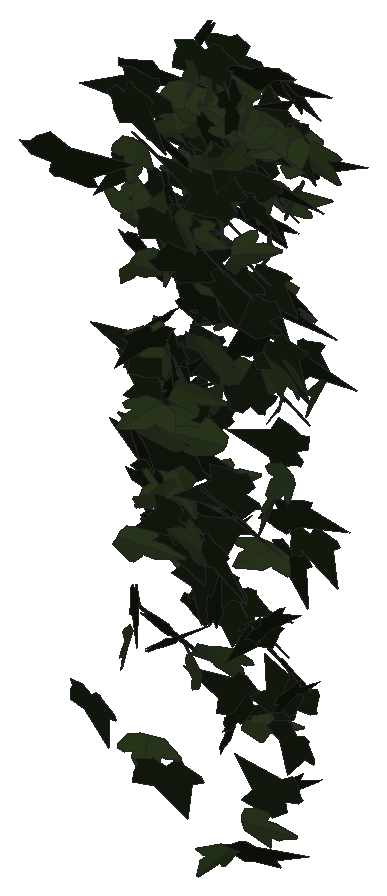
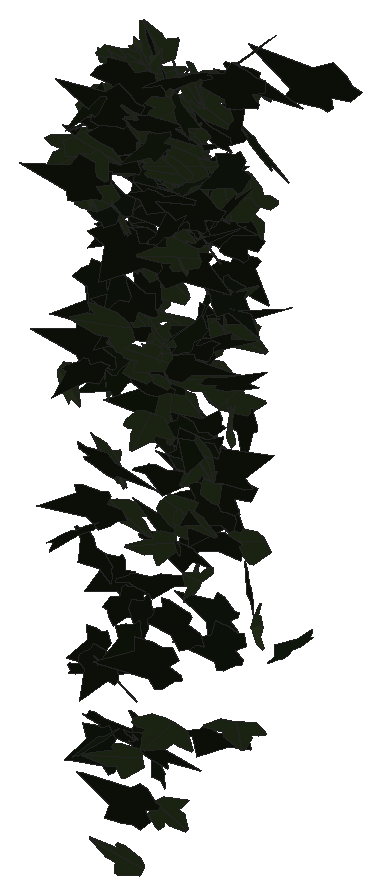
# SketchUp Ruby script. Lengths in millimetres.
U = 1.mm
M = Sketchup.active_model
def pt(a) = Geom::Point3d.new(a.map { |v| v * U })
def face(e, loops, mat)
  f = e.add_face(loops[0].map { |a| pt(a) })
  loops[1..].each { |l| e.add_face(l.map { |a| pt(a) }).erase! }
  f.material = f.back_material = mat if mat
  f
end
# faces: each face lists its corners as indices into pts; further lists are holes
def faces(e, pts, list, mat = nil) = list.each { |f| face(e, (f[0].is_a?(Array) ? f : [f]).map { |l| l.map { |i| pts[i] } }, mat) }
# xy, xz, yz: faces in a plane at the given z, y or x. An outline is a flat list of corners, or four numbers for a rectangle; further outlines are holes
def ring(l) = l.size == 4 ? [[l[0], l[1]], [l[2], l[1]], [l[2], l[3]], [l[0], l[3]]] : l.each_slice(2).to_a
def flat(e, list, mat, &to3) = list.each { |f| face(e, (f[0].is_a?(Array) ? f : [f]).map { |l| ring(l).map { |u, v| to3.(u, v) } }, mat) }
def xy(e, z, list, mat = nil) = flat(e, list, mat) { |x, y| [x, y, z] }
def xz(e, y, list, mat = nil) = flat(e, list, mat) { |x, z| [x, y, z] }
def yz(e, x, list, mat = nil) = flat(e, list, mat) { |y, z| [x, y, z] }
def lines(e, pts, list) = list.each { |a, b| e.add_line(pt(pts[a]), pt(pts[b])) }
# prism: a flat outline (further loops are holes) pulled along v
def prism(e, loops, v, mat = nil)
  f = face(e, loops, mat); d = Geom::Vector3d.new(v.map { |x| x * U })
  f.pushpull(f.normal.samedirection?(d) ? d.length : -d.length)
end
def box(e, o, s, mat = nil) = prism(e, [[o, [o[0] + s[0], o[1], o[2]], [o[0] + s[0], o[1] + s[1], o[2]], [o[0], o[1] + s[1], o[2]]]], [0, 0, s[2]], mat)
def at(x, y, z, deg = 0) = Geom::Transformation.translation(pt([x, y, z])) * Geom::Transformation.rotation(ORIGIN, Z_AXIS, deg.degrees)
def axes(o, x, y, z) = Geom::Transformation.new([*x, 0, *y, 0, *z, 0, *pt(o).to_a, 1])
def part(name) = M.definitions.add(name)
# library, detail: a bought-in or finely detailed component or shape, given as its bounding box
def library(name, o, s) = part(name).tap { |d| box(d.entities, o, s) }
def detail(e, o, s) = box(e.add_group.entities, o, s)
def put(e, d, t, mat = nil) = e.add_instance(d, t).tap { |i| i.material = mat if mat }
def group(e, t, mat = nil) = e.add_group.tap { |g| g.transformation = t; g.material = mat if mat }.entities
root = M.entities
M.materials.add("efeu1").color = [18, 25, 13]
M.materials.add("efeu2").color = [43, 57, 29]
c1 = part("ivyleaf_9")
p = [[39.1,54.8,31.7],[34.5,51.8,30.2],[-5.3,25.2,17.3],[-17.9,28.3,20.9],[-21.6,21.7,17],[-20.2,4.3,5.3],
  [-22.9,-0.3,2.5],[-17.1,-4,-0.6],[-2,-2.1,-1.2],[-0.7,-15.4,-10.1],[16.6,-22.3,-16.7],[21.1,-15.1,-12.5],
  [32.7,-10.7,-11],[46.1,-1.8,-6.6],[30.8,11.2,3.8]]
faces(c1.entities,p,[[0,1,2,3,4,5,6,7,8,9,10,11,12,13,14]],"efeu1")
c2 = part("ivyleaf_10")
p = [[0,12.8,-0.8],[-1.5,51.3,-10.9],[-4.9,51,-11.6],[-13.6,26.5,-7.3],[-13.2,15.9,-4.6],[-21.1,19.3,-7.2],
  [-29.5,16.3,-8.3],[-29.2,8.3,-6.2],[-19.7,-9.8,0.5],[-7.6,-13,4],[1,-12.2,5.8],[-0.4,51.1,-11.1],
  [-1.5,51.1,-10.9],[1,-12.4,5.9],[16.9,-12.4,3.5],[35.1,9.1,-5.1],[35,12.9,-6.1],[20.5,16.4,-4.9],
  [15.8,15,-3.8],[15.3,27.6,-7.1],[12.8,31.3,-7.8]]
faces(c2.entities,p,[[0,1,2,3,4,5,6,7,8,9,10],[11,12,0,13,14,15,16,17,18,19,20]],"efeu2")
put(root,c1,axes([3472.1,793,1622],[-0.35225,-0.18046,-0.9132],[-1.40311,-0.54002,0.25614],[-1.0816,0.75932,-0.03487]))
put(root,c1,axes([3451.8,772.5,1506.4],[-1.43595,0.46546,-0.42029],[0.62665,-0.2656,-0.88522],[-1.01583,-0.8218,0.04804]))
put(root,c2,axes([3421.8,859.5,1058.3],[-0.14393,0.1182,1.04111],[1.12553,-0.85686,0.14023],[1.64618,0.59618,-0.00486]))
put(root,c1,axes([3420.9,714,625.1],[0.19793,-0.92787,0.30072],[0.10417,-0.29639,-0.93345],[1.85342,0.11575,0.02035]))
put(root,c1,axes([3419,841,1495.8],[1.48979,-0.40489,-0.12318],[-0.20728,0.05755,-0.88129],[0.77832,0.79032,0.00107]))
put(root,c2,axes([3427.2,791.4,692.5],[0.34181,-0.37409,0.90819],[0.86577,-0.78658,-0.41396],[1.65679,0.48821,0.02895]))
put(root,c1,axes([3446.5,854.7,1412.6],[-0.36434,-0.24057,0.98515],[-0.90275,-0.86488,-0.30337],[1.70589,-0.50907,0.04986]))
put(root,c1,axes([3442.7,959.7,1644.3],[-0.86292,0.18215,-0.71547],[0.99799,-0.5116,-0.46255],[-0.98914,-0.67509,0.15749]))
put(root,c1,axes([3405,648.6,1545.1],[0.13222,-0.03569,1.15238],[2.04046,-0.42261,-0.07772],[0.80705,1.07434,0.00771]))
put(root,c1,axes([3455.6,781.9,1041.6],[0.91727,-0.17025,-0.85565],[-1.54105,0.27662,-0.51113],[0.61813,0.94229,-0.00455]))
put(root,c2,axes([3440.8,786.4,1418.5],[1.79924,0.10195,-0.02577],[0.04852,0.00397,0.95086],[0.19417,-0.94572,0.00121]))
put(root,c2,axes([3459.5,906.5,1051.1],[1.15014,-0.60497,-0.52342],[-0.65175,0.39721,-0.85447],[1.37596,0.69383,0.03278]))
put(root,c1,axes([3450.8,902.9,1064.1],[0.50747,0.81799,0.29214],[0.15403,0.28087,-0.8603],[-1.64591,0.27849,0.00956]))
put(root,c1,axes([3414.8,862.5,690.6],[1.31175,-0.47271,0.40824],[0.64514,-0.22753,-0.83576],[0.99844,0.76808,0.00367]))
put(root,c1,axes([3480.1,836.1,968.6],[0.39127,-0.112,1.07152],[-1.82011,0.48333,0.23401],[-0.94415,-0.97816,-0.00706]))
put(root,c1,axes([3452.8,976.5,1432.7],[-0.56216,-0.50969,0.66162],[0.75309,0.53261,0.58696],[-1.39979,0.49124,0.05008]))
put(root,c1,axes([3425.8,943.7,1249.7],[0.47858,-0.74354,0.48384],[0.268,-0.46307,-0.7848],[1.66692,0.28792,-0.01273]))
put(root,c1,axes([3414.9,825.1,1621.7],[0.88499,-0.05133,0.75556],[1.4328,-0.06475,-0.46773],[0.15619,0.88482,0.0096]))
put(root,c1,axes([3474.7,820.2,1102.8],[-1.25047,-0.63451,-0.00932],[-0.01096,-0.00745,0.9134],[-1.20768,0.65706,0.00135]))
put(root,c2,axes([3421.9,806.3,847.5],[-0.4665,-0.16136,-0.92547],[1.69703,0.26113,-0.28169],[0.56284,-0.92108,0.08227]))
put(root,c1,axes([3437.2,795.7,766.4],[-0.46223,0.12383,-0.9645],[1.62416,-0.44946,-0.27259],[-0.88726,-0.88726,0.00348]))
put(root,c1,axes([3451.5,901.8,1031.2],[-0.84074,-0.25168,0.71456],[1.18175,0.35361,0.50842],[-0.82604,0.76204,0.00008]))
put(root,c1,axes([3420.4,930.4,1453.5],[0.41714,-0.14525,0.87945],[1.61546,-0.24247,-0.25159],[0.5179,0.87332,0.07642]))
put(root,c2,axes([3456.2,884.2,1011.5],[-0.35114,-0.51425,-0.85622],[0.43905,0.82522,-0.54534],[1.84948,-0.29354,-0.0331]))
put(root,c2,axes([3451.9,974.7,595.6],[-1.63447,-0.09893,-0.32733],[0.61837,0.03983,-0.86448],[0.20293,-0.9182,-0.00224]))
put(root,c2,axes([3454.8,801.4,521.4],[1.43667,0.49216,-0.09203],[-0.14734,-0.04977,-0.90114],[-0.94145,0.75883,0.00059]))
put(root,c1,axes([3471.4,884.9,1370],[0.04755,-0.78714,-0.50493],[0.03315,-0.50463,0.78754],[-1.77951,-0.03043,0.00118]))
put(root,c2,axes([3470.4,836,943.6],[-0.47796,-0.40608,0.90458],[-0.16294,-0.92078,-0.43712],[1.88007,-0.18303,0.19208]))
put(root,c1,axes([3456.2,871,1371.3],[-0.58123,0.7564,0.28371],[0.04531,-0.29475,0.81146],[1.53685,0.29476,0.08337]))
put(root,c2,axes([3465.2,809.5,1397.4],[-1.28858,-0.9214,-0.03429],[-0.0056,-0.04039,1.14321],[-1.75482,0.67672,0.02153]))
put(root,c1,axes([3449.3,919.6,1491.4],[0.22992,-0.88095,0.22752],[0.10537,-0.22197,-0.88887],[1.72843,0.13072,0.02392]))
put(root,c2,axes([3442.8,936.6,1382.9],[0.20751,0.1087,0.91296],[1.09784,0.70781,-0.15317],[-1.36257,0.58685,0.01563]))
put(root,c2,axes([3462.6,923.6,1361.1],[1.0144,-0.74913,-0.00724],[0.01572,-0.00301,0.91938],[-1.42572,-0.53304,0.00499]))
put(root,c1,axes([3497.8,780.3,1191],[-0.87149,-0.83133,-0.32685],[-0.31015,-0.28339,0.94908],[-1.67155,0.48601,-0.00569]))
put(root,c2,axes([3466.2,875.3,795.8],[0.3753,0.516,-0.72589],[0.41139,0.69351,0.5517],[1.64432,-0.29128,0.02765]))
put(root,c1,axes([3471.9,853.8,1394.2],[-1.33431,-0.74002,-0.23058],[0.30808,0.16426,-1.01938],[1.44266,-0.71952,0.00443]))
put(root,c1,axes([3461.9,828,907.5],[0.89835,0.56869,0.60064],[0.68281,0.48236,-0.73864],[-1.41844,0.59237,0.02484]))
put(root,c1,axes([3496.5,973.7,1610.7],[-1.50219,-0.25026,0.31227],[-0.57647,-0.07768,-0.82786],[0.49774,-0.84526,-0.01637]))
put(root,c1,axes([3511.1,964,544.1],[-1.08883,-0.13817,-0.71312],[-1.32084,-0.16401,0.58855],[-0.40813,0.89941,-0.00223]))
put(root,c1,axes([3456.4,977.5,1588.7],[1.25013,-0.51269,-0.28318],[-0.27366,0.27133,-0.82475],[1.08059,0.66184,0.11875]))
put(root,c1,axes([3488.3,789.8,1248],[-0.58696,0.77516,-0.55379],[0.3898,-0.51452,-0.83426],[-1.7707,-0.37022,-0.00008]))
put(root,c1,axes([3443.6,797.7,1339],[0.41083,-0.30888,0.92443],[0.93141,-0.78447,-0.37639],[1.60419,0.53457,-0.0182]))
put(root,c1,axes([3491.7,895.4,1339.6],[-0.00193,0.24337,-0.98585],[-0.07847,-0.98505,-0.24313],[-1.931,0.03979,0.01087]))
put(root,c1,axes([3496.1,824.6,1162.6],[-0.80452,-0.31573,0.75062],[-1.05369,-0.50875,-0.52579],[1.1365,-0.69519,0.04388]))
put(root,c1,axes([3486,809.7,1524],[1.089,-0.74475,0.46475],[-0.49561,0.38579,0.93883],[-1.59555,-0.62814,0.02558]))
put(root,c2,axes([3485.6,906.9,1545],[-0.05226,0.65443,0.5911],[-0.0415,-0.59171,0.65409],[1.67784,0.00575,0.03459]))
put(root,c1,axes([3474,828.9,901],[1.3801,0.61982,-0.03086],[-0.04688,-0.01867,-0.95395],[-1.18018,0.72556,0.00181]))
put(root,c2,axes([3463,961,898.1],[0.03235,-0.05018,-0.93059],[1.1374,0.71476,-0.02763],[1.36097,-0.59615,0.04521]))
put(root,c2,axes([3490.2,912.7,1410.8],[1.3228,-0.55146,-0.36174],[-0.46281,0.27423,-0.88527],[1.16676,0.73399,0.05897]))
put(root,c1,axes([3508.2,896,1158.9],[-0.40564,-0.42032,-0.7923],[-0.53349,-0.74235,0.46923],[-1.62144,0.3494,0.04382]))
put(root,c2,axes([3473.9,752.6,1352.7],[-0.56934,-0.50266,-0.84866],[0.82035,0.73105,-0.58494],[1.68849,-0.52467,-0.00197]))
put(root,c2,axes([3504.5,935.2,1220.5],[0.52954,-0.21537,0.86431],[-1.3157,0.5188,0.35182],[-1.06904,-0.74518,-0.00486]))
put(root,c1,axes([3484.1,923.8,1222.8],[-0.42192,-0.61773,0.64797],[-0.42322,-0.60862,-0.6563],[1.65043,-0.31399,-0.00265]))
put(root,c1,axes([3489,803.2,1464.5],[0.72836,-0.26813,-0.83036],[-1.26472,0.49808,-0.4671],[1.07628,0.76674,0.01305]))
put(root,c1,axes([3477.3,858.6,1032.8],[-0.55077,-0.1796,0.92444],[1.42571,0.54216,0.33984],[-1.08613,0.80274,-0.02269]))
put(root,c2,axes([3496.9,781.1,1216.3],[-0.12586,0.54344,0.78565],[-0.26002,-0.78482,0.53136],[1.79941,-0.07539,0.13174]))
put(root,c2,axes([3483,790.9,938.4],[-0.84604,-0.82706,0.12784],[0.11572,0.11246,0.93895],[-1.58854,0.44867,0.00031]))
put(root,c1,axes([3469,739.4,1638.1],[0.74444,-0.94154,-0.38299],[-0.27324,0.35508,-1.01955],[1.91513,0.41665,0.00341]))
put(root,c2,axes([3520.4,871.1,901.2],[-0.70942,-0.02316,0.83819],[-1.55841,-0.18747,-0.36932],[0.34366,-0.89797,0.05549]))
put(root,c1,axes([3444.3,829.3,927],[0.6763,-0.23544,1.06071],[1.59742,-0.6492,-0.42528],[1.31314,0.911,-0.02894]))
put(root,c2,axes([3485.9,783.9,1054.6],[-1.99103,0.01951,0.22966],[0.43523,-0.04542,1.04556],[0.05478,1.0701,0.04019]))
put(root,c2,axes([3459.2,906.7,1519.4],[0.69793,0.14062,0.84622],[1.32736,0.48695,-0.38315],[-0.95055,0.78323,0.08629]))
put(root,c1,axes([3472.7,845,863.6],[-0.90683,-0.33009,-0.79839],[1.22799,0.47036,-0.57954],[1.09342,-0.80201,-0.01129]))
put(root,c1,axes([3473.7,905.6,1402.5],[1.48046,-0.44693,-0.23945],[-0.36978,0.1423,-0.89676],[0.89133,0.80136,0.02569]))
put(root,c1,axes([3481.2,940.5,1472],[-0.86592,-0.61852,-0.52069],[0.60132,0.41394,-0.7678],[1.41639,-0.55387,0.00764]))
put(root,c2,axes([3505,870.1,879.7],[0.05304,-0.00437,-0.91531],[-0.91449,-0.77948,-0.01091],[-1.48271,0.48061,-0.02601]))
put(root,c2,axes([3515.6,824.8,1574.3],[-0.8509,-0.61172,0.73961],[-0.82835,-0.59798,-0.75769],[1.62808,-0.62396,0.00104]))
put(root,c1,axes([3475.5,797.9,692.6],[0.34244,0.8728,-0.18622],[0.03602,0.18619,0.89095],[1.69811,-0.17996,0.01866]))
put(root,c1,axes([3460.1,965.9,693.1],[1.33731,0.06434,0.59038],[1.12238,0.03219,-0.70541],[-0.13321,0.91719,-0.01665]))
put(root,c2,axes([3513.3,861.8,1476.4],[-0.09066,-0.01804,-0.91004],[-1.21842,-0.64713,0.04634],[-1.23143,0.64162,0.02115]))
put(root,c1,axes([3526.9,875.8,1444.9],[-1.23225,0.34529,0.47022],[-0.82631,0.18399,-0.73293],[-0.74159,-0.77876,0.03533]))
put(root,c1,axes([3462.8,930.8,1444.9],[1.40363,-0.49471,0.29596],[0.46353,-0.16819,-0.88805],[0.99443,0.77667,-0.0038]))
put(root,c2,axes([3505.3,844.2,1636.3],[0.60606,-0.72157,-0.55667],[-0.40953,0.51347,-0.78867],[1.68542,0.38423,0.00854]))
put(root,c2,axes([3472.2,885,1445.5],[1.5058,-0.07752,-0.50345],[0.96452,0.02601,0.79243],[-0.09776,-0.93743,0.06362]))
put(root,c1,axes([3487.4,843.5,1536.7],[-1.24516,0.53903,0.58756],[0.82009,-0.40048,0.84721],[1.27686,0.78287,0.02883]))
put(root,c2,axes([3496.6,878.6,1537],[-0.74562,-0.68563,-0.50952],[0.48997,0.43972,-0.78966],[1.55017,-0.46877,0.00451]))
put(root,c1,axes([3494.5,906,1022.5],[-0.62724,0.92555,0.04367],[0.02648,-0.0414,0.98248],[1.76327,0.32987,0.00078]))
put(root,c2,axes([3505.2,892.3,1090.4],[-0.5695,-1.00001,-0.37227],[0.16506,0.36256,-1.04363],[2.02409,-0.31093,-0.01964]))
put(root,c1,axes([3508.6,919.9,490.5],[0.0511,0.27281,0.86951],[0.29972,0.85541,-0.27325],[-1.7083,0.15824,-0.02193]))
put(root,c2,axes([3507.8,840.5,1333.3],[0.12143,-1.03745,0.12459],[0.00582,-0.12463,-1.0394],[1.98865,0.06371,-0.00457]))
put(root,c1,axes([3514.3,738.3,1257.3],[-0.21622,0.57953,-0.79444],[0.35502,-0.7725,-0.5902],[-1.83754,-0.21744,-0.02055]))
put(root,c2,axes([3501.3,955.6,1091.2],[-0.89499,-0.68373,-0.44092],[0.48793,0.35879,-0.82981],[1.46949,-0.53556,0.00699]))
put(root,c2,axes([3510.6,921.9,1208],[-0.05726,-0.04578,0.92637],[-0.06297,-0.92622,-0.04684],[1.7641,-0.03455,0.0284]))
put(root,c2,axes([3493,902.4,1601.4],[-1.50446,0.02593,-0.4214],[0.80106,-0.02151,-0.79089],[-0.06281,-0.89554,0.00679]))
put(root,c1,axes([3493.1,799.5,493],[-0.63446,-0.6476,-0.54356],[0.47618,0.48255,-0.72836],[1.53704,-0.41681,0.00128]))
put(root,c1,axes([3491.6,893,1649.6],[-0.23988,-1.01416,-0.28006],[0.18337,0.26975,-1.02019],[1.99397,-0.14681,0.06013]))
put(root,c1,axes([3514.6,896.5,1417.8],[0.21009,-0.57035,-0.66871],[0.23863,-0.65685,0.58094],[-1.65562,-0.16705,-0.00113]))
put(root,c2,axes([3501.6,716,1570.2],[1.51618,-0.51106,0.18272],[0.29656,-0.09549,-0.94648],[0.98945,0.81174,0.00369]))
put(root,c1,axes([3519,791.2,922.7],[-0.57672,-0.32577,0.79941],[-0.83181,-0.67272,-0.43982],[1.41678,-0.52757,0.06719]))
put(root,c2,axes([3508.3,831.7,1617.6],[1.23757,0.89956,-0.27856],[-0.35084,-0.21038,-1.10968],[-1.75757,0.6754,0.02537]))
put(root,c1,axes([3515.5,849.3,1388.6],[1.27885,0.09743,-0.58653],[-1.11599,-0.03779,-0.67805],[-0.18714,0.89112,0.03537]))
put(root,c2,axes([3525,731.2,1136.9],[1.01914,0.45469,-0.69958],[-1.06461,-0.42114,-0.70188],[-1.17822,0.77383,0.02908]))
put(root,c1,axes([3477.5,896.5,727.8],[0.25697,-0.0047,-0.9318],[1.70179,0.26557,0.12823],[0.49898,-0.90331,0.04255]))
put(root,c2,axes([3484,912.2,1500.6],[1.03521,-0.13561,-0.83686],[1.58512,-0.10017,0.55757],[-0.30127,-0.99306,0.05804]))
put(root,c2,axes([3491.4,947,1196.2],[0.47382,0.06479,-0.89605],[1.60611,0.30203,0.25631],[0.58641,-0.87958,0.022]))
put(root,c2,axes([3516.8,784.4,1370.2],[1.09888,-0.69903,0.28494],[0.34884,-0.21818,-0.90665],[1.39368,0.60578,0.00227]))
put(root,c2,axes([3557.3,868.8,1526.8],[0.5791,0.05979,-0.98206],[-1.86847,0.08596,-0.29895],[0.12298,1.02451,0.08239]))
put(root,c1,axes([3482.6,854.7,998.8],[1.08815,0.01164,-0.82271],[1.49859,0.28289,0.55122],[0.45428,-0.9611,0.15229]))
put(root,c1,axes([3532.6,918.5,535.4],[-0.80314,0.62784,-0.45369],[-0.57397,0.34272,0.75478],[1.35792,0.5162,0.0507]))
put(root,c1,axes([3510.2,776.5,1434.4],[-0.0815,-0.8497,-0.56476],[0.09102,0.56297,-0.85063],[1.93964,-0.06212,0.01619]))
put(root,c1,axes([3545.9,861.2,1408.2],[-1.22915,0.58215,-0.09351],[0.13312,-0.06207,-0.86948],[-1.11423,-0.64961,-0.00072]))
put(root,c1,axes([3518.6,776.5,1151.3],[0.28519,0.25189,1.10714],[1.10666,0.94216,-0.29306],[-1.85609,0.60045,-0.00462]))
put(root,c1,axes([3511,847,1176.8],[-0.07456,-0.50955,-0.87742],[0.21257,0.87058,-0.51056],[1.91935,-0.11621,0.02246]))
put(root,c2,axes([3517.1,854.5,1620],[1.2651,-0.68417,0.48045],[0.63147,-0.34751,-0.9539],[1.46044,0.74292,-0.00374]))
put(root,c2,axes([3496.6,861.9,1553.2],[1.04427,0.18477,0.81134],[1.42252,0.3177,-0.57783],[-0.69604,0.9265,0.03634]))
put(root,c2,axes([3502.1,778.8,1203.1],[-0.14878,0.06743,1.06056],[1.64322,-0.61598,0.1028],[1.1792,0.86688,-0.00945]))
put(root,c2,axes([3526.5,951.7,1596.8],[1.67257,-0.18659,0.06142],[0.11548,-0.00995,-0.89841],[0.35559,0.88091,0.00286]))
put(root,c2,axes([3519,872.9,1603.8],[1.48686,-0.3259,0.37248],[0.68454,-0.10427,-0.84561],[0.64705,0.85919,0.03867]))
put(root,c2,axes([3511.8,807.8,1397.2],[-1.08252,-0.29266,-0.91905],[1.51329,0.46167,-0.6391],[1.03907,-0.97726,-0.02669]))
put(root,c2,axes([3502.7,788.2,1084.9],[-0.56446,-0.13942,-1.02034],[1.89134,0.23974,-0.32162],[0.51406,-1.03517,0.06294]))
put(root,c1,axes([3520.9,791.9,1208.2],[0.54938,-0.38591,-0.95824],[1.36157,-0.64305,0.47449],[-1.41827,-0.76683,0.08434]))
put(root,c1,axes([3528.9,866.4,849],[-0.14633,0.89712,0.18789],[0.00572,-0.1883,0.90031],[1.74442,0.07587,0.01281]))
put(root,c2,axes([3514.4,800.1,986],[1.04204,-0.25034,0.82787],[1.38422,-0.39694,-0.60105],[0.89075,0.90971,-0.03444]))
put(root,c1,axes([3534.4,941.1,1374.9],[1.83949,0.27053,-0.15593],[-0.28598,-0.04166,-1.00367],[-0.52094,0.97813,0.00038]))
put(root,c2,axes([3525.4,890.3,1130.5],[0.33883,-0.28673,-0.85954],[0.91901,-0.71119,0.33726],[-1.45921,-0.51449,0.01282]))
put(root,c1,axes([3531.2,942.2,703.1],[1.45417,-0.44787,-0.24673],[-0.3856,0.14215,-0.88544],[0.89352,0.79023,0.01944]))
put(root,c1,axes([3570.5,786.6,1287.5],[0.37655,-0.16216,0.92337],[-0.8184,0.82289,0.23665],[-1.58549,-0.46327,0.09715]))
put(root,c2,axes([3544.4,838.9,1532.3],[-0.17512,-0.36241,-0.93936],[0.58513,0.88811,-0.37276],[1.8247,-0.31957,0.02938]))
put(root,c1,axes([3545.5,819.3,1593.5],[0.81087,-0.45107,-0.65872],[-0.87628,0.47115,-0.62042],[1.2413,0.62726,-0.00767]))
put(root,c2,axes([3518.7,863.1,1269.3],[0.44042,-0.21025,-0.99383],[1.42272,-0.65492,0.31261],[-1.30906,-0.78252,0.00539]))
put(root,c1,axes([3553.5,841.9,816.8],[-1.61427,-0.26055,-0.44335],[0.80352,0.13541,-0.88729],[0.55877,-0.94744,-0.00489]))
put(root,c1,axes([3584.3,826.4,1464.8],[-1.26834,-0.74334,-0.28833],[-0.37624,-0.21001,0.99832],[-1.47005,0.69509,-0.00673]))
put(root,c2,axes([3516.9,785.4,1145.5],[-0.54297,-0.09337,1.02708],[1.93938,0.13859,0.29565],[-0.30228,1.05692,0.05196]))
put(root,c2,axes([3528.1,962.5,511.8],[-0.07738,-0.07681,-0.92279],[1.47689,0.50114,-0.0759],[0.96155,-0.77591,0.04232]))
put(root,c2,axes([3522.7,968.4,337.9],[0.2469,-0.0419,-0.87246],[1.54196,-0.32381,0.13602],[-0.62116,-0.82046,-0.00913]))
put(root,c1,axes([3536.1,907.8,1257.6],[0.04499,-0.21488,0.90008],[0.33805,-0.88258,-0.21537],[1.72842,0.17821,0.01869]))
put(root,c1,axes([3529.3,926,731.5],[0.5796,-0.14624,-0.91366],[1.56261,-0.40083,0.33783],[-0.81205,-0.8757,-0.00205]))
put(root,c2,axes([3565.7,840.9,359.2],[-0.42544,-0.67295,0.54403],[-0.2041,-0.53601,-0.70709],[1.63423,-0.24213,0.05332]))
put(root,c2,axes([3565.1,835.5,1405.5],[0.14805,-0.18076,-0.96008],[-0.21675,0.95487,-0.18901],[1.84665,0.12657,0.05479]))
put(root,c1,axes([3554.8,880.3,773],[-0.98627,-0.83814,-0.24813],[0.27427,0.20259,-0.98528],[1.64081,-0.53766,0.01554]))
put(root,c1,axes([3544,939.1,1226.2],[-0.0974,-0.60134,-0.66443],[0.3498,0.64432,-0.5973],[1.66928,-0.17011,0.0864]))
put(root,c1,axes([3564.1,910.7,1638.6],[1.05893,0.71118,-0.20448],[-0.24967,-0.15698,-0.90294],[-1.38604,0.57161,0.00643]))
put(root,c1,axes([3544.5,928.7,1253.7],[1.59945,0.36729,0.12652],[-0.23822,-0.02944,0.91687],[0.6999,-0.84936,0.02294]))
put(root,c1,axes([3550.1,912.2,1428.5],[0.93371,-0.7094,-0.43293],[-0.41179,0.37637,-0.86191],[1.52715,0.53522,0.03228]))
put(root,c1,axes([3602.5,958.5,994.3],[-1.07119,0.31778,0.65359],[-1.07659,0.32745,-0.64633],[-0.86837,-0.79796,-0.00494]))
put(root,c2,axes([3589.1,785,1080],[0.27304,0.2623,0.92207],[-0.94673,-0.77663,0.29832],[1.55966,-0.51734,0.01966]))
put(root,c1,axes([3545.2,934,1545.7],[1.53374,0.55117,0.07252],[-0.16469,-0.00178,0.97519],[1.04514,-0.80913,0.04725]))
put(root,c1,axes([3563.1,831.8,928.7],[-1.06235,-0.56935,-0.43165],[0.56127,0.31533,-0.79728],[1.23856,-0.63124,-0.00895]))
put(root,c2,axes([3568.9,842.2,1283.8],[-0.97383,-0.80094,-0.39216],[0.41997,0.32436,-0.95037],[1.64448,-0.55714,0.01047]))
put(root,c1,axes([3567.1,855.8,1535.2],[-0.77059,-0.86177,0.12051],[-0.06161,-0.11791,-0.95193],[1.65494,-0.40566,0.02068]))
put(root,c2,axes([3572.1,938.9,1416.4],[0.95106,-0.75757,0.09475],[0.11311,-0.0743,-0.90749],[1.44862,0.50316,0.00865]))
put(root,c2,axes([3570.3,772,692.5],[-0.79677,0.68437,0.57434],[0.49206,-0.51433,0.80132],[1.62763,0.4905,0.0389]))
put(root,c1,axes([3543.6,873.8,1556.2],[0.02093,-0.07092,-0.97432],[1.2312,0.73065,-0.04588],[1.39316,-0.64465,0.05518]))
put(root,c2,axes([3547.1,971.5,1243.6],[-0.86134,0.17463,-0.92439],[1.63326,-0.34364,-0.48507],[-0.73355,-0.97017,0.00542]))
put(root,c2,axes([3560.8,751.6,1450.3],[-0.19825,0.22538,-1.01255],[0.7487,-0.93304,-0.24815],[-1.82677,-0.40686,0.00818]))
put(root,c1,axes([3610.8,813.9,1636.1],[-0.26707,0.02184,-1.08873],[-1.90547,0.42913,0.13765],[0.81508,1.01038,-0.03493]))
put(root,c2,axes([3595.2,844.1,1596.3],[-1.01927,0.90235,-0.1716],[-0.2355,0.12595,1.04848],[1.73219,0.54809,0.04157]))
put(root,c2,axes([3584.6,857,1292.8],[0.03798,0.20091,-0.85382],[-0.33471,-0.83578,-0.20077],[-1.63547,0.17572,0.02126]))
put(root,c2,axes([3604.3,835.5,1585.7],[0.76625,0.49015,0.7051],[-0.89315,-0.52658,0.63402],[1.36868,-0.61804,0.01899]))
put(root,c1,axes([3561,741.6,1377.3],[-0.1751,-0.05453,1.03704],[1.90886,0.26521,0.10292],[-0.51233,1.00676,0.02905]))
put(root,c1,axes([3590.2,789.9,785.8],[-0.20763,-0.2453,0.88445],[0.65113,0.81562,0.26841],[-1.62095,0.35905,-0.00547]))
put(root,c1,axes([3564.9,947.6,1420.1],[1.3549,-0.36236,-0.50729],[0.8679,-0.22236,0.79879],[-0.80902,-0.84541,0.00734]))
put(root,c1,axes([3553.3,954.7,1595.4],[0.53239,-0.26078,0.81831],[1.49597,-0.26908,-0.35445],[0.65871,0.82187,0.1436]))
put(root,c2,axes([3597.5,902.1,1347.8],[-0.00335,-0.61601,-0.92274],[-0.01581,0.92272,-0.61598],[2.11148,0.00593,-0.00608]))
put(root,c2,axes([3615.1,845,1185],[-1.26371,-0.45428,0.51951],[-0.76258,-0.3332,-0.80348],[1.06937,-0.77444,0.04095]))
put(root,c1,axes([3601.7,890.5,726.1],[-0.16792,0.2841,-0.87622],[0.45006,-0.84375,-0.29738],[-1.69434,-0.25228,0.00785]))
put(root,c1,axes([3604.4,921.1,1540.6],[-1.48824,-0.30162,0.41554],[0.75659,0.12353,0.83775],[-0.61851,0.87686,0.02491]))
put(root,c1,axes([3593.2,944.6,644.9],[1.44674,-0.16583,-0.50191],[-0.90438,0.17069,-0.77609],[0.44065,0.89478,0.05503]))
put(root,c2,axes([3567.2,887.2,1126.5],[0.75215,-0.30601,-0.93342],[1.34295,-0.61151,0.49924],[-1.3006,-0.80839,-0.02431]))
put(root,c1,axes([3630.1,866.6,1497.4],[-1.47829,0.32028,0.27419],[-0.48572,0.10031,-0.84017],[-0.63871,-0.81758,0.00433]))
put(root,c1,axes([3566.3,784.5,1395],[1.08905,-0.67769,0.5122],[0.63928,-0.38674,-0.88694],[1.48497,0.66349,0.00619]))
put(root,c2,axes([3632.8,696.8,957.5],[-0.27888,0.10602,0.99224],[-1.72475,0.40571,-0.17718],[-0.79508,-0.91729,0.03632]))
put(root,c1,axes([3600.1,924.1,1286.8],[1.57029,0.0021,-0.56346],[-1.06845,0.08855,-0.82173],[0.09176,0.99519,0.07431]))
put(root,c1,axes([3594.7,935.6,1140.2],[1.11529,-0.6927,-0.2414],[0.29462,-0.18524,0.90732],[-1.36467,-0.60611,-0.0014]))
put(root,c2,axes([3633.3,928.3,1509.3],[0.21494,0.00293,-0.93995],[-1.7038,-0.28821,-0.10846],[-0.54524,0.90177,-0.03161]))
put(root,c2,axes([3621,959.2,1527],[0.94978,0.40218,-0.6925],[-1.17586,-0.32577,-0.63443],[-0.96966,0.78897,0.09104]))
put(root,c1,axes([3583.7,918.3,1126.8],[1.44578,-0.52793,-0.14012],[-0.2178,0.08087,-0.92509],[1.01648,0.76823,0.00109]))
put(root,c1,axes([3595.1,954.5,1607.6],[1.18252,-0.43191,-0.50206],[-0.68448,0.35803,-0.75308],[1.0584,0.71409,0.07392]))
put(root,c1,axes([3598.6,968.6,508.8],[-0.2909,-0.77773,0.5064],[-0.13852,-0.5016,-0.79232],[1.76086,-0.16794,0.02133]))
put(root,c2,axes([3585.3,815.5,1201.6],[-0.65633,0.25719,0.93352],[1.43506,-0.55039,0.43018],[1.1562,0.82913,-0.00401]))
put(root,c2,axes([3621.3,875.8,868.9],[1.46967,0.09324,-0.50297],[-0.95593,-0.03437,-0.77751],[-0.18447,0.92093,0.02191]))
put(root,c1,axes([3577.9,936.8,1238.6],[1.52606,-0.15088,0.38349],[0.73082,-0.03099,-0.81509],[0.28471,0.88829,0.03671]))
put(root,c1,axes([3588.2,844.4,1373],[1.58163,-0.52748,-0.44182],[0.74934,-0.20361,0.98366],[-1.07395,-0.9189,0.03566]))
put(root,c1,axes([3602.9,970.3,1154.9],[0.14344,-0.38418,-0.80255],[-0.30964,0.7859,-0.39148],[1.66485,0.17927,-0.00367]))
put(root,c2,axes([3614.3,833.2,1626.7],[0.92268,-0.8241,0.02003],[0.02823,-0.01451,-0.95611],[1.56863,0.485,0.00543]))
put(root,c1,axes([3636.8,911.8,621.7],[-1.53108,0.41023,-0.20214],[0.33163,-0.10322,-0.90295],[-0.80474,-0.82304,0.01249]))
put(root,c1,axes([3588.6,861.8,359.5],[1.22579,0.48312,-0.40607],[0.61856,0.24344,0.80513],[1.0296,-0.72143,-0.00025]))
put(root,c2,axes([3624.2,943.6,1444.3],[0.31541,-0.91126,0.2276],[0.118,-0.22,-0.92597],[1.78369,0.17569,0.02101]))
put(root,c2,axes([3629.9,893.8,1114],[0.14811,-0.75674,-0.58203],[-0.12024,0.5786,-0.76073],[1.81297,0.1002,-0.00291]))
put(root,c2,axes([3620.2,884.2,943.6],[0.64707,-0.76959,0.3817],[0.30039,-0.34756,-0.84134],[1.60712,0.37482,0.00357]))
put(root,c2,axes([3632.1,903.2,981.4],[1.12425,-0.69928,-0.33576],[-0.40365,0.26036,-0.91537],[1.42008,0.62761,0.00563]))
put(root,c1,axes([3642.2,914.2,597.8],[-1.45355,-0.52119,0.25655],[0.42416,0.12845,0.92444],[-1.02099,0.79537,0.01882]))
put(root,c1,axes([3658.3,772.9,1022.1],[-1.66587,0.1588,0.38799],[-0.72589,0.07123,-0.88958],[-0.33123,-0.95478,-0.00184]))
put(root,c1,axes([3624,860.9,752.1],[-0.19506,0.40331,-0.86016],[-0.56037,0.80906,0.41444],[1.71904,0.3095,0.03749]))
put(root,c2,axes([3600.2,937.7,1422.7],[-0.63796,-0.23085,0.82015],[1.27779,0.47106,0.40699],[-0.99837,0.75041,-0.00318]))
put(root,c1,axes([3607.5,946.8,833],[-0.76264,0.0543,-0.94422],[1.78804,-0.09517,-0.40418],[-0.20717,-1.0213,-0.01253]))
put(root,c1,axes([3585.1,886.2,1480.9],[1.00097,-0.45764,0.81289],[1.24994,-0.48107,-0.69575],[1.26085,0.84022,0.04439]))
put(root,c1,axes([3595.1,969.7,1466.2],[0.66549,0.00643,0.87388],[1.64452,0.13813,-0.34677],[-0.24858,0.93105,0.04542]))
put(root,c1,axes([3602.2,933.7,904.9],[0.3241,0.13493,-0.8697],[0.65346,0.80545,0.19219],[1.54228,-0.36962,0.10133]))
put(root,c1,axes([3663.1,819.8,1295.4],[-1.28802,-0.01452,0.65017],[-1.23418,-0.05571,-0.67625],[0.09336,-0.93682,0.03014]))
put(root,c1,axes([3618.5,786.1,1374.9],[-1.30942,-0.34633,-0.68097],[1.17791,0.2846,-0.77005],[0.85245,-0.92525,0.01803]))
put(root,c1,axes([3612.1,857.6,1336.1],[-0.16814,-0.46455,-0.74307],[0.52037,0.69494,-0.46697],[1.58457,-0.27751,0.0745]))
put(root,c1,axes([3663.1,859.2,474.1],[-1.54809,-0.06509,-0.4059],[-0.76521,-0.06147,0.8156],[-0.16297,0.90698,0.02615]))
put(root,c1,axes([3637.8,816.7,1146.8],[-0.87179,-0.38586,0.69445],[1.00131,0.4533,0.5989],[-1.13292,0.69757,-0.00506]))
put(root,c2,axes([3626.7,719.4,1285.2],[-1.59618,0.43825,-0.34025],[0.56376,-0.16775,-0.94622],[-0.89286,-0.88939,0.01081]))
put(root,c2,axes([3639.9,837,1613.8],[1.76613,0.06573,-0.25854],[-0.49299,-0.00163,-0.93016],[-0.12134,0.96332,0.01606]))
put(root,c2,axes([3654.3,893.3,1559.2],[0.58839,0.3457,-0.98261],[-1.25613,-0.72796,-0.46376],[-1.53372,0.72882,0.00286]))
put(root,c2,axes([3621.1,956.5,1508.2],[-1.7179,0.06518,-0.56528],[1.07528,-0.02353,-0.90487],[-0.12893,-1.06478,-0.01461]))
put(root,c1,axes([3627.4,889.4,461.6],[0.65967,0.42746,0.77907],[0.9083,0.61586,-0.55024],[-1.42665,0.58975,0.00992]))
put(root,c1,axes([3624.8,917.4,1552.3],[0.48197,-0.87405,-0.17808],[-0.09691,0.17065,-0.91],[1.6949,0.25831,-0.00139]))
put(root,c2,axes([3655.9,835.4,1602.9],[1.54764,-0.2449,-0.45148],[-0.82826,0.12051,-0.84921],[0.51919,0.92226,-0.00893]))
put(root,c1,axes([3620.5,734.2,940.9],[0.91753,-0.94802,-0.08604],[-0.07485,0.07652,-1.06356],[1.81014,0.4837,-0.00037]))
put(root,c2,axes([3653.2,852.4,1198],[-1.50133,0.53505,0.1537],[-0.26791,0.06618,-0.95288],[-1.02506,-0.80095,0.02394]))
put(root,c1,axes([3610.7,764.2,999.2],[1.61499,-0.64268,0.34444],[0.53858,-0.19681,-1.06439],[1.27897,0.89441,0.01329]))
put(root,c1,axes([3611.3,933,1167.5],[0.6248,0.13811,-0.87175],[1.47147,0.40363,0.35511],[0.81025,-0.83952,0.02732]))
put(root,c1,axes([3634.5,962.5,859.3],[0.1754,-0.86475,-0.31916],[-0.06422,0.31737,-0.86965],[1.75313,0.09814,0.00008]))
put(root,c2,axes([3643.1,753.2,1578.1],[-0.67836,-0.88916,0.14535],[0.1344,0.12826,0.95778],[-1.70944,0.36293,0.01762]))
put(root,c2,axes([3649.5,967.3,1118.9],[0.37925,-0.95291,0.39518],[0.20131,-0.38149,-0.97323],[1.953,0.22437,0.02358]))
put(root,c1,axes([3642.5,883.1,619.3],[0.35908,0.32237,0.85556],[0.91858,0.70682,-0.37276],[-1.47784,0.51767,-0.02382]))
put(root,c1,axes([3633.3,878.6,1215.1],[0.31631,-0.94323,-0.41182],[-0.0571,0.41254,-0.95698],[1.95797,0.16441,0.03862]))
put(root,c2,axes([3653,880.2,1188.2],[-1.37678,0.72719,0.04566],[-0.06786,0.02894,-1.02572],[-1.38506,-0.72426,0.00487]))
put(root,c1,axes([3650.8,780.2,1251.6],[0.91493,0.43756,0.72981],[-1.00341,-0.50478,0.64993],[1.27118,-0.71339,-0.01225]))
put(root,c2,axes([3642.3,784.4,1415.6],[-0.27938,-0.22822,-1.12616],[1.05275,0.98107,-0.27092],[1.91681,-0.57209,-0.01535]))
